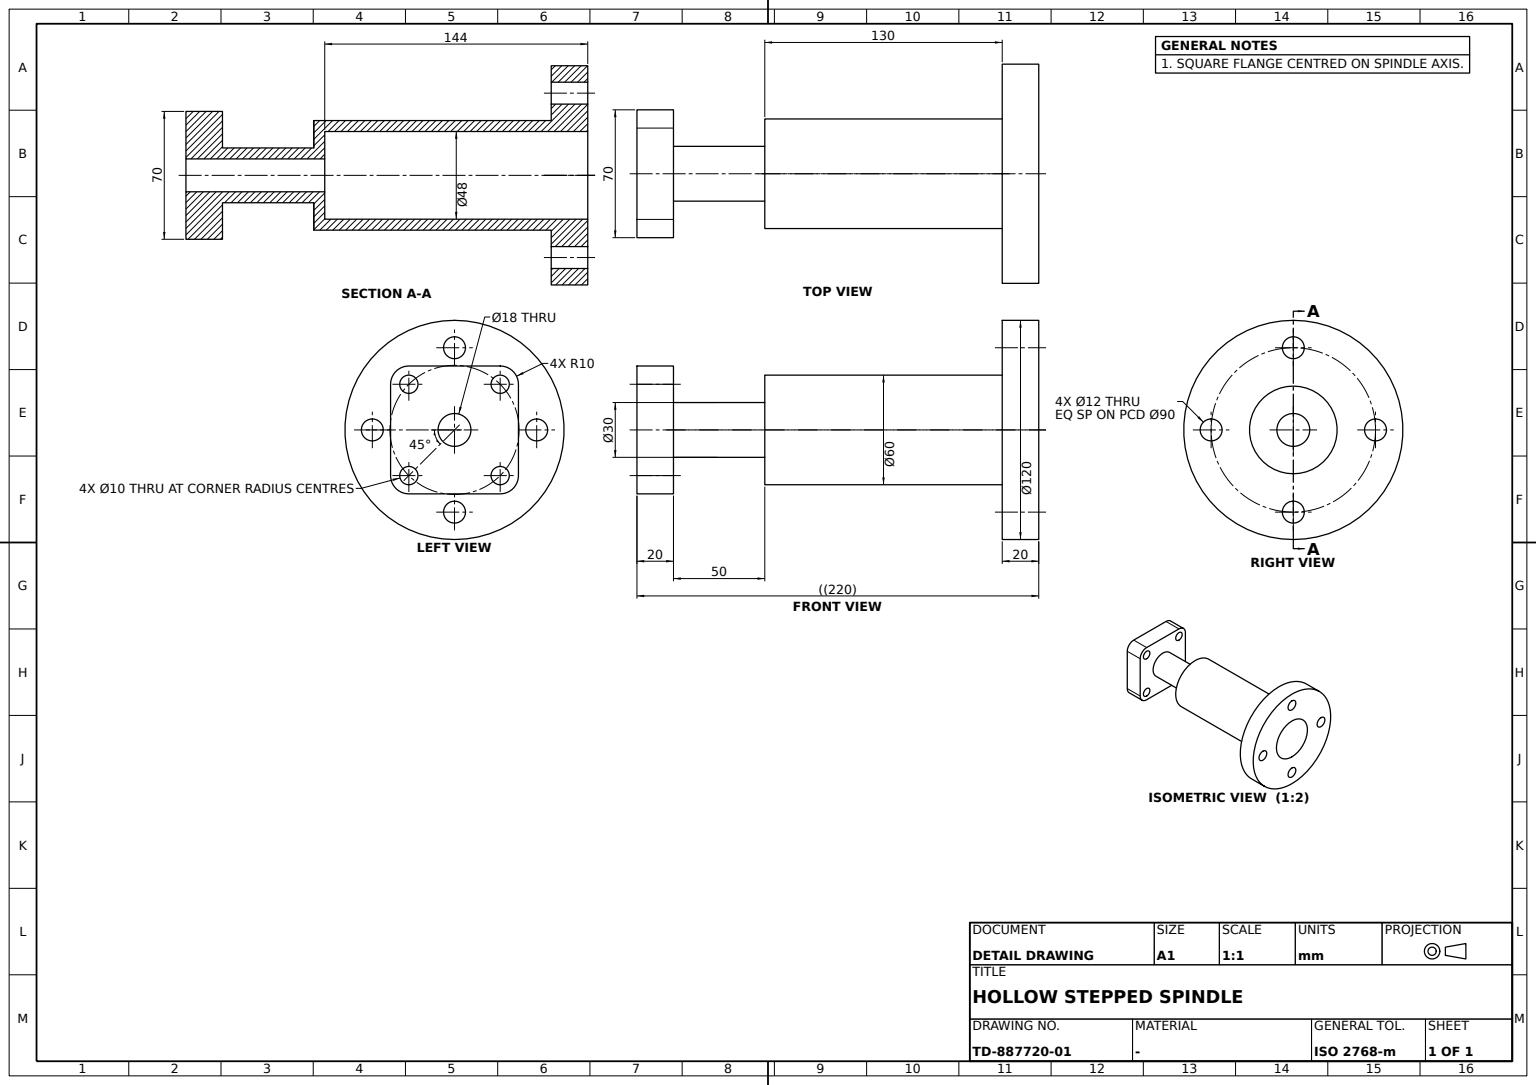
ISO-10303-21;
HEADER;
FILE_DESCRIPTION((''),'2;1');
FILE_NAME('','',(''),(''),'','','');
FILE_SCHEMA(('AUTOMOTIVE_DESIGN'));
ENDSEC;
DATA;
#1=APPLICATION_CONTEXT('');
#2=PRODUCT_CONTEXT('',#1,'mechanical');
#3=PRODUCT('','','',(#2));
#4=PRODUCT_DEFINITION_FORMATION('','',#3);
#5=PRODUCT_DEFINITION_CONTEXT('',#1,'design');
#6=PRODUCT_DEFINITION('','',#4,#5);
#7=PRODUCT_DEFINITION_SHAPE('','',#6);
#8=(LENGTH_UNIT()NAMED_UNIT(*)SI_UNIT(.MILLI.,.METRE.));
#9=(NAMED_UNIT(*)PLANE_ANGLE_UNIT()SI_UNIT($,.RADIAN.));
#10=(NAMED_UNIT(*)SI_UNIT($,.STERADIAN.)SOLID_ANGLE_UNIT());
#11=UNCERTAINTY_MEASURE_WITH_UNIT(LENGTH_MEASURE(0.005),#8,'distance_accuracy_value','');
#12=(GEOMETRIC_REPRESENTATION_CONTEXT(3)GLOBAL_UNCERTAINTY_ASSIGNED_CONTEXT((#11))GLOBAL_UNIT_ASSIGNED_CONTEXT((#8,#9,#10))REPRESENTATION_CONTEXT('',''));
#13=CARTESIAN_POINT('',(-25.,-200.,-35.));
#14=VERTEX_POINT('',#13);
#15=CARTESIAN_POINT('',(-35.,-200.,-25.));
#16=VERTEX_POINT('',#15);
#17=CARTESIAN_POINT('',(-25.,-200.,-25.));
#18=DIRECTION('',(0.,1.,0.));
#19=DIRECTION('',(1.,0.,0.));
#20=AXIS2_PLACEMENT_3D('',#17,#18,#19);
#21=CIRCLE('',#20,10.);
#22=EDGE_CURVE('',#14,#16,#21,.T.);
#23=ORIENTED_EDGE('',*,*,#22,.F.);
#24=CARTESIAN_POINT('',(-25.,-220.,-35.));
#25=VERTEX_POINT('',#24);
#26=VECTOR('',#18,1000.);
#27=LINE('',#24,#26);
#28=EDGE_CURVE('',#25,#14,#27,.T.);
#29=ORIENTED_EDGE('',*,*,#28,.F.);
#30=CARTESIAN_POINT('',(-35.,-220.,-25.));
#31=VERTEX_POINT('',#30);
#32=CARTESIAN_POINT('',(-25.,-220.,-25.));
#33=AXIS2_PLACEMENT_3D('',#32,#18,#19);
#34=CIRCLE('',#33,10.);
#35=EDGE_CURVE('',#25,#31,#34,.T.);
#36=ORIENTED_EDGE('',*,*,#35,.T.);
#37=LINE('',#30,#26);
#38=EDGE_CURVE('',#31,#16,#37,.T.);
#39=ORIENTED_EDGE('',*,*,#38,.T.);
#40=EDGE_LOOP('',(#23,#29,#36,#39));
#41=FACE_BOUND('',#40,.T.);
#42=DIRECTION('',(0.,0.,1.));
#43=AXIS2_PLACEMENT_3D('',#32,#18,#42);
#44=CYLINDRICAL_SURFACE('',#43,10.);
#45=ADVANCED_FACE('',(#41),#44,.T.);
#46=CARTESIAN_POINT('',(0.,0.,-60.));
#47=VERTEX_POINT('',#46);
#48=CARTESIAN_POINT('',(0.,-20.,-60.));
#49=VERTEX_POINT('',#48);
#50=LINE('',#46,#26);
#51=EDGE_CURVE('',#47,#49,#50,.F.);
#52=ORIENTED_EDGE('',*,*,#51,.F.);
#53=CARTESIAN_POINT('',(0.,0.,60.));
#54=VERTEX_POINT('',#53);
#55=CARTESIAN_POINT('',(0.,0.,0.));
#56=AXIS2_PLACEMENT_3D('',#55,#18,#42);
#57=CIRCLE('',#56,60.);
#58=EDGE_CURVE('',#54,#47,#57,.T.);
#59=ORIENTED_EDGE('',*,*,#58,.F.);
#60=CARTESIAN_POINT('',(0.,-20.,60.));
#61=VERTEX_POINT('',#60);
#62=LINE('',#53,#26);
#63=EDGE_CURVE('',#61,#54,#62,.T.);
#64=ORIENTED_EDGE('',*,*,#63,.F.);
#65=CARTESIAN_POINT('',(0.,-20.,0.));
#66=AXIS2_PLACEMENT_3D('',#65,#18,#42);
#67=CIRCLE('',#66,60.);
#68=EDGE_CURVE('',#61,#49,#67,.T.);
#69=ORIENTED_EDGE('',*,*,#68,.T.);
#70=EDGE_LOOP('',(#52,#59,#64,#69));
#71=FACE_BOUND('',#70,.T.);
#72=CYLINDRICAL_SURFACE('',#56,60.);
#73=ADVANCED_FACE('',(#71),#72,.T.);
#74=CARTESIAN_POINT('',(-45.,-20.,6.));
#75=VERTEX_POINT('',#74);
#76=CARTESIAN_POINT('',(-45.,-20.,-6.));
#77=VERTEX_POINT('',#76);
#78=CARTESIAN_POINT('',(-45.,-20.,0.));
#79=DIRECTION('',(0.,-1.,0.));
#80=AXIS2_PLACEMENT_3D('',#78,#79,#19);
#81=CIRCLE('',#80,6.);
#82=EDGE_CURVE('',#75,#77,#81,.T.);
#83=ORIENTED_EDGE('',*,*,#82,.T.);
#84=CARTESIAN_POINT('',(-45.,0.,-6.));
#85=VERTEX_POINT('',#84);
#86=VECTOR('',#79,1000.);
#87=LINE('',#84,#86);
#88=EDGE_CURVE('',#85,#77,#87,.T.);
#89=ORIENTED_EDGE('',*,*,#88,.F.);
#90=CARTESIAN_POINT('',(-45.,0.,6.));
#91=VERTEX_POINT('',#90);
#92=CARTESIAN_POINT('',(-45.,0.,0.));
#93=AXIS2_PLACEMENT_3D('',#92,#79,#19);
#94=CIRCLE('',#93,6.);
#95=EDGE_CURVE('',#91,#85,#94,.T.);
#96=ORIENTED_EDGE('',*,*,#95,.F.);
#97=LINE('',#90,#86);
#98=EDGE_CURVE('',#75,#91,#97,.F.);
#99=ORIENTED_EDGE('',*,*,#98,.F.);
#100=EDGE_LOOP('',(#83,#89,#96,#99));
#101=FACE_BOUND('',#100,.T.);
#102=DIRECTION('',(0.,0.,-1.));
#103=AXIS2_PLACEMENT_3D('',#92,#79,#102);
#104=CYLINDRICAL_SURFACE('',#103,6.);
#105=ADVANCED_FACE('',(#101),#104,.F.);
#106=CARTESIAN_POINT('',(25.,-200.,20.));
#107=VERTEX_POINT('',#106);
#108=CARTESIAN_POINT('',(25.,-200.,30.));
#109=VERTEX_POINT('',#108);
#110=CARTESIAN_POINT('',(25.,-200.,25.));
#111=AXIS2_PLACEMENT_3D('',#110,#18,#42);
#112=CIRCLE('',#111,5.);
#113=EDGE_CURVE('',#107,#109,#112,.T.);
#114=ORIENTED_EDGE('',*,*,#113,.T.);
#115=CARTESIAN_POINT('',(25.,-220.,30.));
#116=VERTEX_POINT('',#115);
#117=LINE('',#115,#26);
#118=EDGE_CURVE('',#109,#116,#117,.F.);
#119=ORIENTED_EDGE('',*,*,#118,.T.);
#120=CARTESIAN_POINT('',(25.,-220.,20.));
#121=VERTEX_POINT('',#120);
#122=CARTESIAN_POINT('',(25.,-220.,25.));
#123=AXIS2_PLACEMENT_3D('',#122,#18,#42);
#124=CIRCLE('',#123,5.);
#125=EDGE_CURVE('',#121,#116,#124,.T.);
#126=ORIENTED_EDGE('',*,*,#125,.F.);
#127=LINE('',#120,#26);
#128=EDGE_CURVE('',#121,#107,#127,.T.);
#129=ORIENTED_EDGE('',*,*,#128,.T.);
#130=EDGE_LOOP('',(#114,#119,#126,#129));
#131=FACE_BOUND('',#130,.T.);
#132=CYLINDRICAL_SURFACE('',#123,5.);
#133=ADVANCED_FACE('',(#131),#132,.F.);
#134=CARTESIAN_POINT('',(0.,-20.,30.));
#135=VERTEX_POINT('',#134);
#136=CARTESIAN_POINT('',(0.,-150.,30.));
#137=VERTEX_POINT('',#136);
#138=CARTESIAN_POINT('',(0.,0.,30.));
#139=LINE('',#138,#26);
#140=EDGE_CURVE('',#135,#137,#139,.F.);
#141=ORIENTED_EDGE('',*,*,#140,.F.);
#142=CARTESIAN_POINT('',(0.,-20.,-30.));
#143=VERTEX_POINT('',#142);
#144=CIRCLE('',#66,30.);
#145=EDGE_CURVE('',#143,#135,#144,.T.);
#146=ORIENTED_EDGE('',*,*,#145,.F.);
#147=CARTESIAN_POINT('',(0.,-150.,-30.));
#148=VERTEX_POINT('',#147);
#149=CARTESIAN_POINT('',(0.,0.,-30.));
#150=LINE('',#149,#26);
#151=EDGE_CURVE('',#148,#143,#150,.T.);
#152=ORIENTED_EDGE('',*,*,#151,.F.);
#153=CARTESIAN_POINT('',(0.,-150.,0.));
#154=AXIS2_PLACEMENT_3D('',#153,#18,#42);
#155=CIRCLE('',#154,30.);
#156=EDGE_CURVE('',#148,#137,#155,.T.);
#157=ORIENTED_EDGE('',*,*,#156,.T.);
#158=EDGE_LOOP('',(#141,#146,#152,#157));
#159=FACE_BOUND('',#158,.T.);
#160=CYLINDRICAL_SURFACE('',#56,30.);
#161=ADVANCED_FACE('',(#159),#160,.T.);
#162=EDGE_CURVE('',#109,#107,#112,.T.);
#163=ORIENTED_EDGE('',*,*,#162,.F.);
#164=ORIENTED_EDGE('',*,*,#113,.F.);
#165=EDGE_LOOP('',(#163,#164));
#166=FACE_BOUND('',#165,.T.);
#167=CARTESIAN_POINT('',(-25.,-200.,20.));
#168=VERTEX_POINT('',#167);
#169=CARTESIAN_POINT('',(-25.,-200.,30.));
#170=VERTEX_POINT('',#169);
#171=CARTESIAN_POINT('',(-25.,-200.,25.));
#172=DIRECTION('',(-1.,0.,0.));
#173=AXIS2_PLACEMENT_3D('',#171,#18,#172);
#174=CIRCLE('',#173,5.);
#175=EDGE_CURVE('',#168,#170,#174,.T.);
#176=ORIENTED_EDGE('',*,*,#175,.F.);
#177=EDGE_CURVE('',#170,#168,#174,.T.);
#178=ORIENTED_EDGE('',*,*,#177,.F.);
#179=EDGE_LOOP('',(#176,#178));
#180=FACE_BOUND('',#179,.T.);
#181=CARTESIAN_POINT('',(-25.,-200.,-30.));
#182=VERTEX_POINT('',#181);
#183=CARTESIAN_POINT('',(-25.,-200.,-20.));
#184=VERTEX_POINT('',#183);
#185=AXIS2_PLACEMENT_3D('',#17,#18,#102);
#186=CIRCLE('',#185,5.);
#187=EDGE_CURVE('',#182,#184,#186,.T.);
#188=ORIENTED_EDGE('',*,*,#187,.F.);
#189=EDGE_CURVE('',#184,#182,#186,.T.);
#190=ORIENTED_EDGE('',*,*,#189,.F.);
#191=EDGE_LOOP('',(#188,#190));
#192=FACE_BOUND('',#191,.T.);
#193=CARTESIAN_POINT('',(25.,-200.,-20.));
#194=VERTEX_POINT('',#193);
#195=CARTESIAN_POINT('',(25.,-200.,-30.));
#196=VERTEX_POINT('',#195);
#197=CARTESIAN_POINT('',(25.,-200.,-25.));
#198=AXIS2_PLACEMENT_3D('',#197,#18,#19);
#199=CIRCLE('',#198,5.);
#200=EDGE_CURVE('',#194,#196,#199,.T.);
#201=ORIENTED_EDGE('',*,*,#200,.F.);
#202=EDGE_CURVE('',#196,#194,#199,.T.);
#203=ORIENTED_EDGE('',*,*,#202,.F.);
#204=EDGE_LOOP('',(#201,#203));
#205=FACE_BOUND('',#204,.T.);
#206=CARTESIAN_POINT('',(0.,-200.,15.));
#207=VERTEX_POINT('',#206);
#208=CARTESIAN_POINT('',(0.,-200.,-15.));
#209=VERTEX_POINT('',#208);
#210=CARTESIAN_POINT('',(0.,-200.,0.));
#211=AXIS2_PLACEMENT_3D('',#210,#18,#42);
#212=CIRCLE('',#211,15.);
#213=EDGE_CURVE('',#207,#209,#212,.T.);
#214=ORIENTED_EDGE('',*,*,#213,.F.);
#215=EDGE_CURVE('',#209,#207,#212,.T.);
#216=ORIENTED_EDGE('',*,*,#215,.F.);
#217=EDGE_LOOP('',(#214,#216));
#218=FACE_BOUND('',#217,.T.);
#219=CARTESIAN_POINT('',(-35.,-200.,25.));
#220=VERTEX_POINT('',#219);
#221=VECTOR('',#42,1000.);
#222=LINE('',#15,#221);
#223=EDGE_CURVE('',#16,#220,#222,.T.);
#224=ORIENTED_EDGE('',*,*,#223,.T.);
#225=CARTESIAN_POINT('',(-25.,-200.,35.));
#226=VERTEX_POINT('',#225);
#227=AXIS2_PLACEMENT_3D('',#171,#18,#19);
#228=CIRCLE('',#227,10.);
#229=EDGE_CURVE('',#220,#226,#228,.T.);
#230=ORIENTED_EDGE('',*,*,#229,.T.);
#231=CARTESIAN_POINT('',(25.,-200.,35.));
#232=VERTEX_POINT('',#231);
#233=VECTOR('',#19,1000.);
#234=LINE('',#225,#233);
#235=EDGE_CURVE('',#226,#232,#234,.T.);
#236=ORIENTED_EDGE('',*,*,#235,.T.);
#237=CARTESIAN_POINT('',(35.,-200.,25.));
#238=VERTEX_POINT('',#237);
#239=AXIS2_PLACEMENT_3D('',#110,#18,#19);
#240=CIRCLE('',#239,10.);
#241=EDGE_CURVE('',#232,#238,#240,.T.);
#242=ORIENTED_EDGE('',*,*,#241,.T.);
#243=CARTESIAN_POINT('',(35.,-200.,-25.));
#244=VERTEX_POINT('',#243);
#245=VECTOR('',#102,1000.);
#246=LINE('',#237,#245);
#247=EDGE_CURVE('',#238,#244,#246,.T.);
#248=ORIENTED_EDGE('',*,*,#247,.T.);
#249=CARTESIAN_POINT('',(25.,-200.,-35.));
#250=VERTEX_POINT('',#249);
#251=CIRCLE('',#198,10.);
#252=EDGE_CURVE('',#244,#250,#251,.T.);
#253=ORIENTED_EDGE('',*,*,#252,.T.);
#254=VECTOR('',#172,1000.);
#255=LINE('',#249,#254);
#256=EDGE_CURVE('',#250,#14,#255,.T.);
#257=ORIENTED_EDGE('',*,*,#256,.T.);
#258=ORIENTED_EDGE('',*,*,#22,.T.);
#259=EDGE_LOOP('',(#224,#230,#236,#242,#248,#253,#257,#258));
#260=FACE_BOUND('',#259,.T.);
#261=AXIS2_PLACEMENT_3D('',#206,#18,#42);
#262=PLANE('',#261);
#263=ADVANCED_FACE('',(#166,#180,#192,#205,#218,#260),#262,.T.);
#264=CARTESIAN_POINT('',(45.,-20.,6.));
#265=VERTEX_POINT('',#264);
#266=CARTESIAN_POINT('',(45.,-20.,-6.));
#267=VERTEX_POINT('',#266);
#268=CARTESIAN_POINT('',(45.,-20.,0.));
#269=AXIS2_PLACEMENT_3D('',#268,#79,#19);
#270=CIRCLE('',#269,6.);
#271=EDGE_CURVE('',#265,#267,#270,.T.);
#272=ORIENTED_EDGE('',*,*,#271,.F.);
#273=EDGE_CURVE('',#267,#265,#270,.T.);
#274=ORIENTED_EDGE('',*,*,#273,.F.);
#275=EDGE_LOOP('',(#272,#274));
#276=FACE_BOUND('',#275,.T.);
#277=EDGE_CURVE('',#49,#61,#67,.T.);
#278=ORIENTED_EDGE('',*,*,#277,.F.);
#279=ORIENTED_EDGE('',*,*,#68,.F.);
#280=EDGE_LOOP('',(#278,#279));
#281=FACE_BOUND('',#280,.T.);
#282=EDGE_CURVE('',#77,#75,#81,.T.);
#283=ORIENTED_EDGE('',*,*,#282,.F.);
#284=ORIENTED_EDGE('',*,*,#82,.F.);
#285=EDGE_LOOP('',(#283,#284));
#286=FACE_BOUND('',#285,.T.);
#287=CARTESIAN_POINT('',(0.,-20.,39.));
#288=VERTEX_POINT('',#287);
#289=CARTESIAN_POINT('',(0.,-20.,51.));
#290=VERTEX_POINT('',#289);
#291=CARTESIAN_POINT('',(0.,-20.,45.));
#292=AXIS2_PLACEMENT_3D('',#291,#79,#19);
#293=CIRCLE('',#292,6.);
#294=EDGE_CURVE('',#288,#290,#293,.T.);
#295=ORIENTED_EDGE('',*,*,#294,.F.);
#296=EDGE_CURVE('',#290,#288,#293,.T.);
#297=ORIENTED_EDGE('',*,*,#296,.F.);
#298=EDGE_LOOP('',(#295,#297));
#299=FACE_BOUND('',#298,.T.);
#300=CARTESIAN_POINT('',(0.,-20.,-39.));
#301=VERTEX_POINT('',#300);
#302=CARTESIAN_POINT('',(0.,-20.,-51.));
#303=VERTEX_POINT('',#302);
#304=CARTESIAN_POINT('',(0.,-20.,-45.));
#305=AXIS2_PLACEMENT_3D('',#304,#79,#19);
#306=CIRCLE('',#305,6.);
#307=EDGE_CURVE('',#301,#303,#306,.T.);
#308=ORIENTED_EDGE('',*,*,#307,.F.);
#309=EDGE_CURVE('',#303,#301,#306,.T.);
#310=ORIENTED_EDGE('',*,*,#309,.F.);
#311=EDGE_LOOP('',(#308,#310));
#312=FACE_BOUND('',#311,.T.);
#313=EDGE_CURVE('',#135,#143,#144,.T.);
#314=ORIENTED_EDGE('',*,*,#313,.T.);
#315=ORIENTED_EDGE('',*,*,#145,.T.);
#316=EDGE_LOOP('',(#314,#315));
#317=FACE_BOUND('',#316,.T.);
#318=AXIS2_PLACEMENT_3D('',#60,#79,#102);
#319=PLANE('',#318);
#320=ADVANCED_FACE('',(#276,#281,#286,#299,#312,#317),#319,.T.);
#321=CARTESIAN_POINT('',(25.,-220.,-35.));
#322=VERTEX_POINT('',#321);
#323=LINE('',#321,#26);
#324=EDGE_CURVE('',#322,#250,#323,.T.);
#325=ORIENTED_EDGE('',*,*,#324,.T.);
#326=ORIENTED_EDGE('',*,*,#252,.F.);
#327=CARTESIAN_POINT('',(35.,-220.,-25.));
#328=VERTEX_POINT('',#327);
#329=LINE('',#327,#26);
#330=EDGE_CURVE('',#328,#244,#329,.T.);
#331=ORIENTED_EDGE('',*,*,#330,.F.);
#332=CARTESIAN_POINT('',(25.,-220.,-25.));
#333=AXIS2_PLACEMENT_3D('',#332,#18,#19);
#334=CIRCLE('',#333,10.);
#335=EDGE_CURVE('',#328,#322,#334,.T.);
#336=ORIENTED_EDGE('',*,*,#335,.T.);
#337=EDGE_LOOP('',(#325,#326,#331,#336));
#338=FACE_BOUND('',#337,.T.);
#339=AXIS2_PLACEMENT_3D('',#332,#18,#42);
#340=CYLINDRICAL_SURFACE('',#339,10.);
#341=ADVANCED_FACE('',(#338),#340,.T.);
#342=ORIENTED_EDGE('',*,*,#213,.T.);
#343=CARTESIAN_POINT('',(0.,-150.,-15.));
#344=VERTEX_POINT('',#343);
#345=CARTESIAN_POINT('',(0.,0.,-15.));
#346=LINE('',#345,#26);
#347=EDGE_CURVE('',#209,#344,#346,.T.);
#348=ORIENTED_EDGE('',*,*,#347,.T.);
#349=CARTESIAN_POINT('',(0.,-150.,15.));
#350=VERTEX_POINT('',#349);
#351=CIRCLE('',#154,15.);
#352=EDGE_CURVE('',#350,#344,#351,.T.);
#353=ORIENTED_EDGE('',*,*,#352,.F.);
#354=CARTESIAN_POINT('',(0.,0.,15.));
#355=LINE('',#354,#26);
#356=EDGE_CURVE('',#350,#207,#355,.F.);
#357=ORIENTED_EDGE('',*,*,#356,.T.);
#358=EDGE_LOOP('',(#342,#348,#353,#357));
#359=FACE_BOUND('',#358,.T.);
#360=CYLINDRICAL_SURFACE('',#56,15.);
#361=ADVANCED_FACE('',(#359),#360,.T.);
#362=CARTESIAN_POINT('',(0.,-144.,24.));
#363=VERTEX_POINT('',#362);
#364=CARTESIAN_POINT('',(0.,-144.,-24.));
#365=VERTEX_POINT('',#364);
#366=CARTESIAN_POINT('',(0.,-144.,0.));
#367=AXIS2_PLACEMENT_3D('',#366,#18,#42);
#368=CIRCLE('',#367,24.);
#369=EDGE_CURVE('',#363,#365,#368,.T.);
#370=ORIENTED_EDGE('',*,*,#369,.F.);
#371=CARTESIAN_POINT('',(0.,0.,24.));
#372=VERTEX_POINT('',#371);
#373=LINE('',#371,#26);
#374=EDGE_CURVE('',#363,#372,#373,.T.);
#375=ORIENTED_EDGE('',*,*,#374,.T.);
#376=CARTESIAN_POINT('',(0.,0.,-24.));
#377=VERTEX_POINT('',#376);
#378=CIRCLE('',#56,24.);
#379=EDGE_CURVE('',#372,#377,#378,.T.);
#380=ORIENTED_EDGE('',*,*,#379,.T.);
#381=LINE('',#376,#26);
#382=EDGE_CURVE('',#377,#365,#381,.F.);
#383=ORIENTED_EDGE('',*,*,#382,.T.);
#384=EDGE_LOOP('',(#370,#375,#380,#383));
#385=FACE_BOUND('',#384,.T.);
#386=CYLINDRICAL_SURFACE('',#56,24.);
#387=ADVANCED_FACE('',(#385),#386,.F.);
#388=ORIENTED_EDGE('',*,*,#313,.F.);
#389=ORIENTED_EDGE('',*,*,#140,.T.);
#390=EDGE_CURVE('',#137,#148,#155,.T.);
#391=ORIENTED_EDGE('',*,*,#390,.T.);
#392=ORIENTED_EDGE('',*,*,#151,.T.);
#393=EDGE_LOOP('',(#388,#389,#391,#392));
#394=FACE_BOUND('',#393,.T.);
#395=ADVANCED_FACE('',(#394),#160,.T.);
#396=ORIENTED_EDGE('',*,*,#202,.T.);
#397=CARTESIAN_POINT('',(25.,-220.,-20.));
#398=VERTEX_POINT('',#397);
#399=LINE('',#397,#26);
#400=EDGE_CURVE('',#398,#194,#399,.T.);
#401=ORIENTED_EDGE('',*,*,#400,.F.);
#402=CARTESIAN_POINT('',(25.,-220.,-30.));
#403=VERTEX_POINT('',#402);
#404=CIRCLE('',#333,5.);
#405=EDGE_CURVE('',#403,#398,#404,.T.);
#406=ORIENTED_EDGE('',*,*,#405,.F.);
#407=LINE('',#402,#26);
#408=EDGE_CURVE('',#196,#403,#407,.F.);
#409=ORIENTED_EDGE('',*,*,#408,.F.);
#410=EDGE_LOOP('',(#396,#401,#406,#409));
#411=FACE_BOUND('',#410,.T.);
#412=CYLINDRICAL_SURFACE('',#339,5.);
#413=ADVANCED_FACE('',(#411),#412,.F.);
#414=ORIENTED_EDGE('',*,*,#156,.F.);
#415=ORIENTED_EDGE('',*,*,#390,.F.);
#416=EDGE_LOOP('',(#414,#415));
#417=FACE_BOUND('',#416,.T.);
#418=ORIENTED_EDGE('',*,*,#352,.T.);
#419=EDGE_CURVE('',#344,#350,#351,.T.);
#420=ORIENTED_EDGE('',*,*,#419,.T.);
#421=EDGE_LOOP('',(#418,#420));
#422=FACE_BOUND('',#421,.T.);
#423=AXIS2_PLACEMENT_3D('',#136,#79,#102);
#424=PLANE('',#423);
#425=ADVANCED_FACE('',(#417,#422),#424,.T.);
#426=ORIENTED_EDGE('',*,*,#28,.T.);
#427=ORIENTED_EDGE('',*,*,#256,.F.);
#428=ORIENTED_EDGE('',*,*,#324,.F.);
#429=LINE('',#321,#254);
#430=EDGE_CURVE('',#322,#25,#429,.T.);
#431=ORIENTED_EDGE('',*,*,#430,.T.);
#432=EDGE_LOOP('',(#426,#427,#428,#431));
#433=FACE_BOUND('',#432,.T.);
#434=AXIS2_PLACEMENT_3D('',#321,#102,#172);
#435=PLANE('',#434);
#436=ADVANCED_FACE('',(#433),#435,.T.);
#437=CARTESIAN_POINT('',(-25.,-220.,-20.));
#438=VERTEX_POINT('',#437);
#439=CARTESIAN_POINT('',(-25.,-220.,-30.));
#440=VERTEX_POINT('',#439);
#441=AXIS2_PLACEMENT_3D('',#32,#18,#102);
#442=CIRCLE('',#441,5.);
#443=EDGE_CURVE('',#438,#440,#442,.T.);
#444=ORIENTED_EDGE('',*,*,#443,.T.);
#445=EDGE_CURVE('',#440,#438,#442,.T.);
#446=ORIENTED_EDGE('',*,*,#445,.T.);
#447=EDGE_LOOP('',(#444,#446));
#448=FACE_BOUND('',#447,.T.);
#449=ORIENTED_EDGE('',*,*,#125,.T.);
#450=EDGE_CURVE('',#116,#121,#124,.T.);
#451=ORIENTED_EDGE('',*,*,#450,.T.);
#452=EDGE_LOOP('',(#449,#451));
#453=FACE_BOUND('',#452,.T.);
#454=EDGE_CURVE('',#398,#403,#404,.T.);
#455=ORIENTED_EDGE('',*,*,#454,.T.);
#456=ORIENTED_EDGE('',*,*,#405,.T.);
#457=EDGE_LOOP('',(#455,#456));
#458=FACE_BOUND('',#457,.T.);
#459=CARTESIAN_POINT('',(25.,-220.,35.));
#460=VERTEX_POINT('',#459);
#461=CARTESIAN_POINT('',(35.,-220.,25.));
#462=VERTEX_POINT('',#461);
#463=AXIS2_PLACEMENT_3D('',#122,#18,#19);
#464=CIRCLE('',#463,10.);
#465=EDGE_CURVE('',#460,#462,#464,.T.);
#466=ORIENTED_EDGE('',*,*,#465,.F.);
#467=CARTESIAN_POINT('',(-25.,-220.,35.));
#468=VERTEX_POINT('',#467);
#469=LINE('',#467,#233);
#470=EDGE_CURVE('',#468,#460,#469,.T.);
#471=ORIENTED_EDGE('',*,*,#470,.F.);
#472=CARTESIAN_POINT('',(-35.,-220.,25.));
#473=VERTEX_POINT('',#472);
#474=CARTESIAN_POINT('',(-25.,-220.,25.));
#475=AXIS2_PLACEMENT_3D('',#474,#18,#19);
#476=CIRCLE('',#475,10.);
#477=EDGE_CURVE('',#473,#468,#476,.T.);
#478=ORIENTED_EDGE('',*,*,#477,.F.);
#479=LINE('',#30,#221);
#480=EDGE_CURVE('',#31,#473,#479,.T.);
#481=ORIENTED_EDGE('',*,*,#480,.F.);
#482=ORIENTED_EDGE('',*,*,#35,.F.);
#483=ORIENTED_EDGE('',*,*,#430,.F.);
#484=ORIENTED_EDGE('',*,*,#335,.F.);
#485=LINE('',#461,#245);
#486=EDGE_CURVE('',#462,#328,#485,.T.);
#487=ORIENTED_EDGE('',*,*,#486,.F.);
#488=EDGE_LOOP('',(#466,#471,#478,#481,#482,#483,#484,#487));
#489=FACE_BOUND('',#488,.T.);
#490=CARTESIAN_POINT('',(-25.,-220.,30.));
#491=VERTEX_POINT('',#490);
#492=CARTESIAN_POINT('',(-25.,-220.,20.));
#493=VERTEX_POINT('',#492);
#494=AXIS2_PLACEMENT_3D('',#474,#18,#172);
#495=CIRCLE('',#494,5.);
#496=EDGE_CURVE('',#491,#493,#495,.T.);
#497=ORIENTED_EDGE('',*,*,#496,.T.);
#498=EDGE_CURVE('',#493,#491,#495,.T.);
#499=ORIENTED_EDGE('',*,*,#498,.T.);
#500=EDGE_LOOP('',(#497,#499));
#501=FACE_BOUND('',#500,.T.);
#502=CARTESIAN_POINT('',(0.,-220.,-9.));
#503=VERTEX_POINT('',#502);
#504=CARTESIAN_POINT('',(0.,-220.,9.));
#505=VERTEX_POINT('',#504);
#506=CARTESIAN_POINT('',(0.,-220.,0.));
#507=AXIS2_PLACEMENT_3D('',#506,#18,#42);
#508=CIRCLE('',#507,9.);
#509=EDGE_CURVE('',#503,#505,#508,.T.);
#510=ORIENTED_EDGE('',*,*,#509,.T.);
#511=EDGE_CURVE('',#505,#503,#508,.T.);
#512=ORIENTED_EDGE('',*,*,#511,.T.);
#513=EDGE_LOOP('',(#510,#512));
#514=FACE_BOUND('',#513,.T.);
#515=CARTESIAN_POINT('',(0.,-220.,35.));
#516=AXIS2_PLACEMENT_3D('',#515,#79,#102);
#517=PLANE('',#516);
#518=ADVANCED_FACE('',(#448,#453,#458,#489,#501,#514),#517,.T.);
#519=CARTESIAN_POINT('',(45.,0.,-6.));
#520=VERTEX_POINT('',#519);
#521=LINE('',#519,#86);
#522=EDGE_CURVE('',#267,#520,#521,.F.);
#523=ORIENTED_EDGE('',*,*,#522,.F.);
#524=ORIENTED_EDGE('',*,*,#273,.T.);
#525=CARTESIAN_POINT('',(45.,0.,6.));
#526=VERTEX_POINT('',#525);
#527=LINE('',#525,#86);
#528=EDGE_CURVE('',#526,#265,#527,.T.);
#529=ORIENTED_EDGE('',*,*,#528,.F.);
#530=CARTESIAN_POINT('',(45.,0.,0.));
#531=AXIS2_PLACEMENT_3D('',#530,#79,#19);
#532=CIRCLE('',#531,6.);
#533=EDGE_CURVE('',#520,#526,#532,.T.);
#534=ORIENTED_EDGE('',*,*,#533,.F.);
#535=EDGE_LOOP('',(#523,#524,#529,#534));
#536=FACE_BOUND('',#535,.T.);
#537=AXIS2_PLACEMENT_3D('',#530,#79,#102);
#538=CYLINDRICAL_SURFACE('',#537,6.);
#539=ADVANCED_FACE('',(#536),#538,.F.);
#540=ORIENTED_EDGE('',*,*,#177,.T.);
#541=LINE('',#492,#26);
#542=EDGE_CURVE('',#493,#168,#541,.T.);
#543=ORIENTED_EDGE('',*,*,#542,.F.);
#544=ORIENTED_EDGE('',*,*,#496,.F.);
#545=LINE('',#490,#26);
#546=EDGE_CURVE('',#170,#491,#545,.F.);
#547=ORIENTED_EDGE('',*,*,#546,.F.);
#548=EDGE_LOOP('',(#540,#543,#544,#547));
#549=FACE_BOUND('',#548,.T.);
#550=AXIS2_PLACEMENT_3D('',#474,#18,#42);
#551=CYLINDRICAL_SURFACE('',#550,5.);
#552=ADVANCED_FACE('',(#549),#551,.F.);
#553=EDGE_CURVE('',#526,#520,#532,.T.);
#554=ORIENTED_EDGE('',*,*,#553,.T.);
#555=ORIENTED_EDGE('',*,*,#533,.T.);
#556=EDGE_LOOP('',(#554,#555));
#557=FACE_BOUND('',#556,.T.);
#558=CARTESIAN_POINT('',(0.,0.,-51.));
#559=VERTEX_POINT('',#558);
#560=CARTESIAN_POINT('',(0.,0.,-39.));
#561=VERTEX_POINT('',#560);
#562=CARTESIAN_POINT('',(0.,0.,-45.));
#563=AXIS2_PLACEMENT_3D('',#562,#79,#19);
#564=CIRCLE('',#563,6.);
#565=EDGE_CURVE('',#559,#561,#564,.T.);
#566=ORIENTED_EDGE('',*,*,#565,.T.);
#567=EDGE_CURVE('',#561,#559,#564,.T.);
#568=ORIENTED_EDGE('',*,*,#567,.T.);
#569=EDGE_LOOP('',(#566,#568));
#570=FACE_BOUND('',#569,.T.);
#571=CARTESIAN_POINT('',(0.,0.,39.));
#572=VERTEX_POINT('',#571);
#573=CARTESIAN_POINT('',(0.,0.,51.));
#574=VERTEX_POINT('',#573);
#575=CARTESIAN_POINT('',(0.,0.,45.));
#576=AXIS2_PLACEMENT_3D('',#575,#79,#19);
#577=CIRCLE('',#576,6.);
#578=EDGE_CURVE('',#572,#574,#577,.T.);
#579=ORIENTED_EDGE('',*,*,#578,.T.);
#580=EDGE_CURVE('',#574,#572,#577,.T.);
#581=ORIENTED_EDGE('',*,*,#580,.T.);
#582=EDGE_LOOP('',(#579,#581));
#583=FACE_BOUND('',#582,.T.);
#584=EDGE_CURVE('',#377,#372,#378,.T.);
#585=ORIENTED_EDGE('',*,*,#584,.F.);
#586=ORIENTED_EDGE('',*,*,#379,.F.);
#587=EDGE_LOOP('',(#585,#586));
#588=FACE_BOUND('',#587,.T.);
#589=ORIENTED_EDGE('',*,*,#58,.T.);
#590=EDGE_CURVE('',#47,#54,#57,.T.);
#591=ORIENTED_EDGE('',*,*,#590,.T.);
#592=EDGE_LOOP('',(#589,#591));
#593=FACE_BOUND('',#592,.T.);
#594=EDGE_CURVE('',#85,#91,#94,.T.);
#595=ORIENTED_EDGE('',*,*,#594,.T.);
#596=ORIENTED_EDGE('',*,*,#95,.T.);
#597=EDGE_LOOP('',(#595,#596));
#598=FACE_BOUND('',#597,.T.);
#599=AXIS2_PLACEMENT_3D('',#371,#18,#42);
#600=PLANE('',#599);
#601=ADVANCED_FACE('',(#557,#570,#583,#588,#593,#598),#600,.T.);
#602=ORIENTED_EDGE('',*,*,#546,.T.);
#603=ORIENTED_EDGE('',*,*,#498,.F.);
#604=ORIENTED_EDGE('',*,*,#542,.T.);
#605=ORIENTED_EDGE('',*,*,#175,.T.);
#606=EDGE_LOOP('',(#602,#603,#604,#605));
#607=FACE_BOUND('',#606,.T.);
#608=ADVANCED_FACE('',(#607),#551,.F.);
#609=ORIENTED_EDGE('',*,*,#223,.F.);
#610=ORIENTED_EDGE('',*,*,#38,.F.);
#611=ORIENTED_EDGE('',*,*,#480,.T.);
#612=LINE('',#472,#26);
#613=EDGE_CURVE('',#473,#220,#612,.T.);
#614=ORIENTED_EDGE('',*,*,#613,.T.);
#615=EDGE_LOOP('',(#609,#610,#611,#614));
#616=FACE_BOUND('',#615,.T.);
#617=AXIS2_PLACEMENT_3D('',#30,#172,#42);
#618=PLANE('',#617);
#619=ADVANCED_FACE('',(#616),#618,.T.);
#620=CARTESIAN_POINT('',(0.,-144.,9.));
#621=VERTEX_POINT('',#620);
#622=CARTESIAN_POINT('',(0.,-144.,-9.));
#623=VERTEX_POINT('',#622);
#624=CIRCLE('',#367,9.);
#625=EDGE_CURVE('',#621,#623,#624,.T.);
#626=ORIENTED_EDGE('',*,*,#625,.T.);
#627=CARTESIAN_POINT('',(0.,0.,-9.));
#628=LINE('',#627,#26);
#629=EDGE_CURVE('',#623,#503,#628,.F.);
#630=ORIENTED_EDGE('',*,*,#629,.T.);
#631=ORIENTED_EDGE('',*,*,#511,.F.);
#632=CARTESIAN_POINT('',(0.,0.,9.));
#633=LINE('',#632,#26);
#634=EDGE_CURVE('',#505,#621,#633,.T.);
#635=ORIENTED_EDGE('',*,*,#634,.T.);
#636=EDGE_LOOP('',(#626,#630,#631,#635));
#637=FACE_BOUND('',#636,.T.);
#638=CYLINDRICAL_SURFACE('',#56,9.);
#639=ADVANCED_FACE('',(#637),#638,.F.);
#640=ORIENTED_EDGE('',*,*,#509,.F.);
#641=ORIENTED_EDGE('',*,*,#629,.F.);
#642=EDGE_CURVE('',#623,#621,#624,.T.);
#643=ORIENTED_EDGE('',*,*,#642,.T.);
#644=ORIENTED_EDGE('',*,*,#634,.F.);
#645=EDGE_LOOP('',(#640,#641,#643,#644));
#646=FACE_BOUND('',#645,.T.);
#647=ADVANCED_FACE('',(#646),#638,.F.);
#648=LINE('',#439,#26);
#649=EDGE_CURVE('',#440,#182,#648,.T.);
#650=ORIENTED_EDGE('',*,*,#649,.F.);
#651=ORIENTED_EDGE('',*,*,#443,.F.);
#652=LINE('',#437,#26);
#653=EDGE_CURVE('',#184,#438,#652,.F.);
#654=ORIENTED_EDGE('',*,*,#653,.F.);
#655=ORIENTED_EDGE('',*,*,#189,.T.);
#656=EDGE_LOOP('',(#650,#651,#654,#655));
#657=FACE_BOUND('',#656,.T.);
#658=CYLINDRICAL_SURFACE('',#43,5.);
#659=ADVANCED_FACE('',(#657),#658,.F.);
#660=LINE('',#571,#86);
#661=EDGE_CURVE('',#288,#572,#660,.F.);
#662=ORIENTED_EDGE('',*,*,#661,.T.);
#663=ORIENTED_EDGE('',*,*,#580,.F.);
#664=LINE('',#573,#86);
#665=EDGE_CURVE('',#574,#290,#664,.T.);
#666=ORIENTED_EDGE('',*,*,#665,.T.);
#667=ORIENTED_EDGE('',*,*,#296,.T.);
#668=EDGE_LOOP('',(#662,#663,#666,#667));
#669=FACE_BOUND('',#668,.T.);
#670=AXIS2_PLACEMENT_3D('',#575,#79,#102);
#671=CYLINDRICAL_SURFACE('',#670,6.);
#672=ADVANCED_FACE('',(#669),#671,.F.);
#673=ORIENTED_EDGE('',*,*,#450,.F.);
#674=ORIENTED_EDGE('',*,*,#118,.F.);
#675=ORIENTED_EDGE('',*,*,#162,.T.);
#676=ORIENTED_EDGE('',*,*,#128,.F.);
#677=EDGE_LOOP('',(#673,#674,#675,#676));
#678=FACE_BOUND('',#677,.T.);
#679=ADVANCED_FACE('',(#678),#132,.F.);
#680=ORIENTED_EDGE('',*,*,#400,.T.);
#681=ORIENTED_EDGE('',*,*,#200,.T.);
#682=ORIENTED_EDGE('',*,*,#408,.T.);
#683=ORIENTED_EDGE('',*,*,#454,.F.);
#684=EDGE_LOOP('',(#680,#681,#682,#683));
#685=FACE_BOUND('',#684,.T.);
#686=ADVANCED_FACE('',(#685),#412,.F.);
#687=ORIENTED_EDGE('',*,*,#229,.F.);
#688=ORIENTED_EDGE('',*,*,#613,.F.);
#689=ORIENTED_EDGE('',*,*,#477,.T.);
#690=LINE('',#467,#26);
#691=EDGE_CURVE('',#468,#226,#690,.T.);
#692=ORIENTED_EDGE('',*,*,#691,.T.);
#693=EDGE_LOOP('',(#687,#688,#689,#692));
#694=FACE_BOUND('',#693,.T.);
#695=CYLINDRICAL_SURFACE('',#550,10.);
#696=ADVANCED_FACE('',(#694),#695,.T.);
#697=ORIENTED_EDGE('',*,*,#356,.F.);
#698=ORIENTED_EDGE('',*,*,#419,.F.);
#699=ORIENTED_EDGE('',*,*,#347,.F.);
#700=ORIENTED_EDGE('',*,*,#215,.T.);
#701=EDGE_LOOP('',(#697,#698,#699,#700));
#702=FACE_BOUND('',#701,.T.);
#703=ADVANCED_FACE('',(#702),#360,.T.);
#704=ORIENTED_EDGE('',*,*,#470,.T.);
#705=LINE('',#459,#26);
#706=EDGE_CURVE('',#460,#232,#705,.T.);
#707=ORIENTED_EDGE('',*,*,#706,.T.);
#708=ORIENTED_EDGE('',*,*,#235,.F.);
#709=ORIENTED_EDGE('',*,*,#691,.F.);
#710=EDGE_LOOP('',(#704,#707,#708,#709));
#711=FACE_BOUND('',#710,.T.);
#712=AXIS2_PLACEMENT_3D('',#467,#42,#19);
#713=PLANE('',#712);
#714=ADVANCED_FACE('',(#711),#713,.T.);
#715=ORIENTED_EDGE('',*,*,#307,.T.);
#716=LINE('',#558,#86);
#717=EDGE_CURVE('',#303,#559,#716,.F.);
#718=ORIENTED_EDGE('',*,*,#717,.T.);
#719=ORIENTED_EDGE('',*,*,#567,.F.);
#720=LINE('',#560,#86);
#721=EDGE_CURVE('',#561,#301,#720,.T.);
#722=ORIENTED_EDGE('',*,*,#721,.T.);
#723=EDGE_LOOP('',(#715,#718,#719,#722));
#724=FACE_BOUND('',#723,.T.);
#725=AXIS2_PLACEMENT_3D('',#562,#79,#102);
#726=CYLINDRICAL_SURFACE('',#725,6.);
#727=ADVANCED_FACE('',(#724),#726,.F.);
#728=ORIENTED_EDGE('',*,*,#187,.T.);
#729=ORIENTED_EDGE('',*,*,#653,.T.);
#730=ORIENTED_EDGE('',*,*,#445,.F.);
#731=ORIENTED_EDGE('',*,*,#649,.T.);
#732=EDGE_LOOP('',(#728,#729,#730,#731));
#733=FACE_BOUND('',#732,.T.);
#734=ADVANCED_FACE('',(#733),#658,.F.);
#735=LINE('',#461,#26);
#736=EDGE_CURVE('',#462,#238,#735,.T.);
#737=ORIENTED_EDGE('',*,*,#736,.F.);
#738=ORIENTED_EDGE('',*,*,#486,.T.);
#739=ORIENTED_EDGE('',*,*,#330,.T.);
#740=ORIENTED_EDGE('',*,*,#247,.F.);
#741=EDGE_LOOP('',(#737,#738,#739,#740));
#742=FACE_BOUND('',#741,.T.);
#743=AXIS2_PLACEMENT_3D('',#461,#19,#102);
#744=PLANE('',#743);
#745=ADVANCED_FACE('',(#742),#744,.T.);
#746=ORIENTED_EDGE('',*,*,#382,.F.);
#747=ORIENTED_EDGE('',*,*,#584,.T.);
#748=ORIENTED_EDGE('',*,*,#374,.F.);
#749=EDGE_CURVE('',#365,#363,#368,.T.);
#750=ORIENTED_EDGE('',*,*,#749,.F.);
#751=EDGE_LOOP('',(#746,#747,#748,#750));
#752=FACE_BOUND('',#751,.T.);
#753=ADVANCED_FACE('',(#752),#386,.F.);
#754=ORIENTED_EDGE('',*,*,#528,.T.);
#755=ORIENTED_EDGE('',*,*,#271,.T.);
#756=ORIENTED_EDGE('',*,*,#522,.T.);
#757=ORIENTED_EDGE('',*,*,#553,.F.);
#758=EDGE_LOOP('',(#754,#755,#756,#757));
#759=FACE_BOUND('',#758,.T.);
#760=ADVANCED_FACE('',(#759),#538,.F.);
#761=ORIENTED_EDGE('',*,*,#465,.T.);
#762=ORIENTED_EDGE('',*,*,#736,.T.);
#763=ORIENTED_EDGE('',*,*,#241,.F.);
#764=ORIENTED_EDGE('',*,*,#706,.F.);
#765=EDGE_LOOP('',(#761,#762,#763,#764));
#766=FACE_BOUND('',#765,.T.);
#767=CYLINDRICAL_SURFACE('',#123,10.);
#768=ADVANCED_FACE('',(#766),#767,.T.);
#769=ORIENTED_EDGE('',*,*,#369,.T.);
#770=ORIENTED_EDGE('',*,*,#749,.T.);
#771=EDGE_LOOP('',(#769,#770));
#772=FACE_BOUND('',#771,.T.);
#773=ORIENTED_EDGE('',*,*,#625,.F.);
#774=ORIENTED_EDGE('',*,*,#642,.F.);
#775=EDGE_LOOP('',(#773,#774));
#776=FACE_BOUND('',#775,.T.);
#777=AXIS2_PLACEMENT_3D('',#620,#18,#42);
#778=PLANE('',#777);
#779=ADVANCED_FACE('',(#772,#776),#778,.T.);
#780=ORIENTED_EDGE('',*,*,#282,.T.);
#781=ORIENTED_EDGE('',*,*,#98,.T.);
#782=ORIENTED_EDGE('',*,*,#594,.F.);
#783=ORIENTED_EDGE('',*,*,#88,.T.);
#784=EDGE_LOOP('',(#780,#781,#782,#783));
#785=FACE_BOUND('',#784,.T.);
#786=ADVANCED_FACE('',(#785),#104,.F.);
#787=ORIENTED_EDGE('',*,*,#578,.F.);
#788=ORIENTED_EDGE('',*,*,#661,.F.);
#789=ORIENTED_EDGE('',*,*,#294,.T.);
#790=ORIENTED_EDGE('',*,*,#665,.F.);
#791=EDGE_LOOP('',(#787,#788,#789,#790));
#792=FACE_BOUND('',#791,.T.);
#793=ADVANCED_FACE('',(#792),#671,.F.);
#794=ORIENTED_EDGE('',*,*,#309,.T.);
#795=ORIENTED_EDGE('',*,*,#721,.F.);
#796=ORIENTED_EDGE('',*,*,#565,.F.);
#797=ORIENTED_EDGE('',*,*,#717,.F.);
#798=EDGE_LOOP('',(#794,#795,#796,#797));
#799=FACE_BOUND('',#798,.T.);
#800=ADVANCED_FACE('',(#799),#726,.F.);
#801=ORIENTED_EDGE('',*,*,#63,.T.);
#802=ORIENTED_EDGE('',*,*,#590,.F.);
#803=ORIENTED_EDGE('',*,*,#51,.T.);
#804=ORIENTED_EDGE('',*,*,#277,.T.);
#805=EDGE_LOOP('',(#801,#802,#803,#804));
#806=FACE_BOUND('',#805,.T.);
#807=ADVANCED_FACE('',(#806),#72,.T.);
#808=CLOSED_SHELL('',(#45,#73,#105,#133,#161,#263,#320,#341,#361,#387,#395,#413,#425,#436,#518,#539,#552,#601,#608,#619,#639,#647,#659,#672,#679,#686,#696,#703,#714,#727,#734,#745,#753,#760,#768,#779,#786,#793,#800,#807));
#809=MANIFOLD_SOLID_BREP('',#808);
#810=ADVANCED_BREP_SHAPE_REPRESENTATION('',(#809),#12);
#811=SHAPE_DEFINITION_REPRESENTATION(#7,#810);
ENDSEC;
END-ISO-10303-21;
